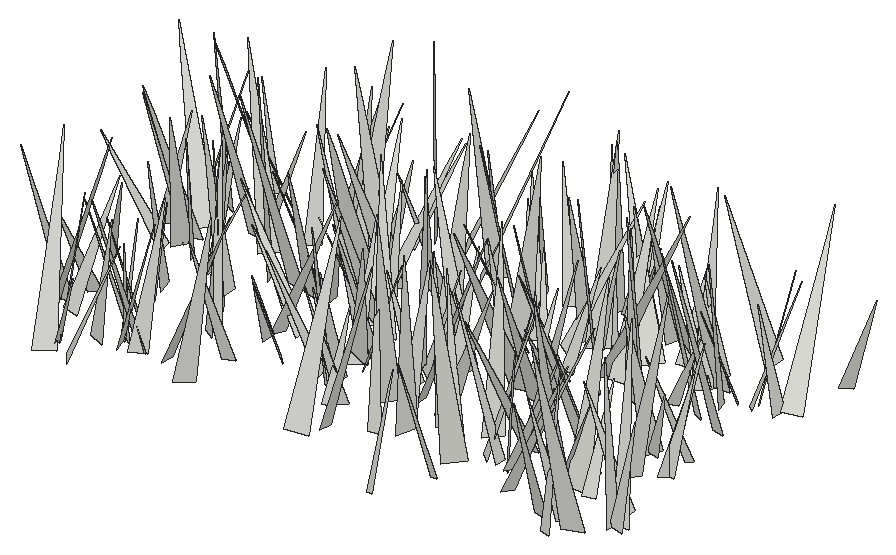
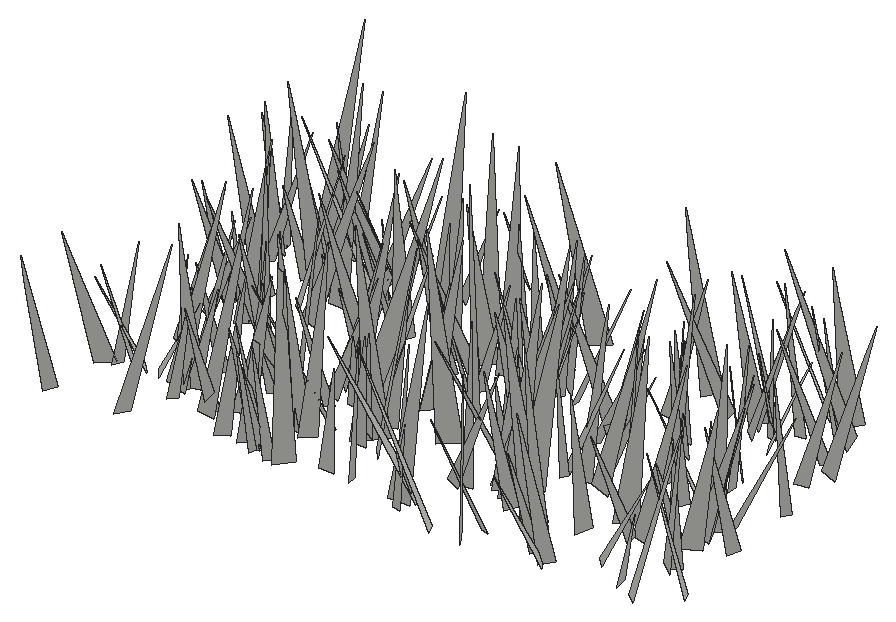
# SketchUp Ruby script. Lengths in inches.
U = 1.inch
M = Sketchup.active_model
def pt(a) = Geom::Point3d.new(a.map { |v| v * U })
def face(e, loops, mat)
  f = e.add_face(loops[0].map { |a| pt(a) })
  loops[1..].each { |l| e.add_face(l.map { |a| pt(a) }).erase! }
  f.material = f.back_material = mat if mat
  f
end
# faces: each face lists its corners as indices into pts; further lists are holes
def faces(e, pts, list, mat = nil) = list.each { |f| face(e, (f[0].is_a?(Array) ? f : [f]).map { |l| l.map { |i| pts[i] } }, mat) }
# xy, xz, yz: faces in a plane at the given z, y or x. An outline is a flat list of corners, or four numbers for a rectangle; further outlines are holes
def ring(l) = l.size == 4 ? [[l[0], l[1]], [l[2], l[1]], [l[2], l[3]], [l[0], l[3]]] : l.each_slice(2).to_a
def flat(e, list, mat, &to3) = list.each { |f| face(e, (f[0].is_a?(Array) ? f : [f]).map { |l| ring(l).map { |u, v| to3.(u, v) } }, mat) }
def xy(e, z, list, mat = nil) = flat(e, list, mat) { |x, y| [x, y, z] }
def xz(e, y, list, mat = nil) = flat(e, list, mat) { |x, z| [x, y, z] }
def yz(e, x, list, mat = nil) = flat(e, list, mat) { |y, z| [x, y, z] }
def lines(e, pts, list) = list.each { |a, b| e.add_line(pt(pts[a]), pt(pts[b])) }
# prism: a flat outline (further loops are holes) pulled along v
def prism(e, loops, v, mat = nil)
  f = face(e, loops, mat); d = Geom::Vector3d.new(v.map { |x| x * U })
  f.pushpull(f.normal.samedirection?(d) ? d.length : -d.length)
end
def box(e, o, s, mat = nil) = prism(e, [[o, [o[0] + s[0], o[1], o[2]], [o[0] + s[0], o[1] + s[1], o[2]], [o[0], o[1] + s[1], o[2]]]], [0, 0, s[2]], mat)
def at(x, y, z, deg = 0) = Geom::Transformation.translation(pt([x, y, z])) * Geom::Transformation.rotation(ORIGIN, Z_AXIS, deg.degrees)
def axes(o, x, y, z) = Geom::Transformation.new([*x, 0, *y, 0, *z, 0, *pt(o).to_a, 1])
def part(name) = M.definitions.add(name)
# library, detail: a bought-in or finely detailed component or shape, given as its bounding box
def library(name, o, s) = part(name).tap { |d| box(d.entities, o, s) }
def detail(e, o, s) = box(e.add_group.entities, o, s)
def put(e, d, t, mat = nil) = e.add_instance(d, t).tap { |i| i.material = mat if mat }
def group(e, t, mat = nil) = e.add_group.tap { |g| g.transformation = t; g.material = mat if mat }.entities
root = M.entities
c1 = part("fur_instance\#9")
p = [[0.8125,0,1.79],[0.67,-0.02,1.48],[0,-0.11,0],[0,0.11,0]]
faces(c1.entities,p,[[0,1,2,3]])
put(root,c1,axes([532.74,130.88,-21.66],[1.96135,3.70682,0.36248],[3.45553,-1.96392,1.38604],[-1.38968,0.34826,3.95807]))
put(root,c1,axes([503.99,133.75,-21.66],[3.91302,0.34843,0.25725],[0.41449,-3.69091,-1.30566],[-0.12562,-1.32482,3.70519]))
put(root,c1,axes([505.79,132.53,-21.66],[4.04604,3.23344,0.3968],[3.2461,-3.94826,-0.92578],[0.27467,-0.96906,5.09593]))
put(root,c1,axes([546.5,135.29,-21.66],[1.61042,-7.88282,1.5376],[-7.97737,-1.75156,-0.62458],[-0.92985,1.37466,8.02136]))
put(root,c1,axes([543.62,135.5,-21.66],[-0.77388,-5.77446,0.46112],[-5.72229,0.83441,0.84559],[0.90132,0.33953,5.76439]))
put(root,c1,axes([503.95,132.42,-21.66],[-5.29033,5.65073,1.03717],[5.57546,5.38985,-0.92613],[1.38587,-0.11308,7.68509]))
put(root,c1,axes([513.87,134.89,-21.66],[5.12868,-4.19399,1.94705],[-4.5125,-5.17419,0.74098],[-1.00889,1.82269,6.58361]))
put(root,c1,axes([545.2,135.82,-21.66],[0.47741,-4.86513,1.33169],[-4.92648,-0.73691,-0.92606],[-1.08291,1.20759,4.79999]))
put(root,c1,axes([534.81,135.12,-21.66],[0.7235,3.49331,2.20248],[3.65755,-1.58024,1.30491],[-1.91742,-1.69623,3.32022]))
put(root,c1,axes([505.73,135.68,-21.66],[-0.80392,-5.00028,1.94874],[-5.12712,1.2977,1.21465],[1.58527,1.66129,4.91668]))
put(root,c1,axes([503.87,134.27,-21.66],[4.42151,2.80893,1.55928],[2.73673,-4.68252,0.67492],[-1.68278,-0.23477,5.19464]))
put(root,c1,axes([545.27,133.86,-21.66],[2.35955,4.93164,1.36493],[4.86886,-2.62618,1.07189],[-1.57426,-0.73054,5.36093]))
put(root,c1,axes([502.5,134.3125,-21.66],[7.43833,2.19546,1.23858],[2.06036,-7.51855,0.95355],[-1.45225,0.57818,7.69672]))
put(root,c1,axes([509.09,136.38,-21.66],[-2.70694,-4.99144,1.16007],[-5.08628,2.45713,-1.29614],[-0.62448,1.62351,5.52829]))
put(root,c1,axes([507.4,136.17,-21.66],[5.27684,1.71083,0.85913],[1.8324,-5.24307,-0.81398],[-0.55438,-1.04563,5.4872]))
put(root,c1,axes([523.9,134.1875,-21.66],[-2.77927,7.20298,1.80131],[7.21654,3.07297,-1.15349],[1.74623,-1.2353,7.63392]))
put(root,c1,axes([507.19,137.08,-21.66],[-1.65671,-3.63214,1.3485],[-3.6613,1.94738,0.7471],[1.26719,0.87797,3.92161]))
put(root,c1,axes([534.58,137.59,-21.66],[4.88048,-6.02987,2.56967],[-6.14977,-5.32095,-0.80587],[-2.26779,1.4525,7.7155]))
put(root,c1,axes([508.95,136.0625,-21.66],[3.9195,-3.82723,2.46639],[-4.43668,-3.94163,0.93419],[-1.02305,2.43088,5.39791]))
put(root,c1,axes([548.6875,137.11,-21.66],[0.22976,-4.49295,1.68417],[-4.67204,0.17468,1.10336],[1.09322,1.69077,4.36142]))
put(root,c1,axes([524.9375,135.9375,-21.66],[6.05583,0.88682,1.38397],[0.67013,-6.15634,1.01257],[-1.50092,0.82941,6.03608]))
put(root,c1,axes([508.51,137.63,-21.66],[-2.89225,-3.68575,0.79235],[-3.76683,2.78458,-0.79678],[-0.15371,1.11313,4.61682]))
put(root,c1,axes([511.09,136.54,-21.66],[6.06997,0.80019,0.53139],[0.73411,-6.05703,0.73529],[-0.61948,0.66277,6.07817]))
put(root,c1,axes([539.79,136.8125,-21.66],[5.54197,-0.978,0.47716],[-1.05474,-5.437,1.10644],[-0.26776,1.17482,5.51777]))
put(root,c1,axes([514.28,139.09,-21.66],[0.3349,-5.08877,0.86463],[-5.08924,-0.4702,-0.79617],[-0.86188,0.79915,5.03725]))
put(root,c1,axes([529.61,138.8,-21.66],[6.66168,-2.88093,2.18206],[-2.80757,-7.00677,-0.67958],[-2.27567,0.211,7.22605]))
put(root,c1,axes([500.96,138.7,-21.66],[-1.48365,-5.76059,1.44193],[-5.8771,1.21156,-1.20691],[-0.85046,1.67706,5.82486]))
put(root,c1,axes([548.28,137.3,-21.66],[-5.81537,-0.03657,1.70774],[-0.23888,6.01751,-0.6846],[1.69135,0.72416,5.77505]))
put(root,c1,axes([507.2,136.69,-21.66],[1.88548,3.67223,0.79609],[3.49899,-2.04056,1.12569],[-1.36969,-0.15771,3.97154]))
put(root,c1,axes([523.89,139.15,-21.66],[0.22156,-4.52657,1.23949],[-4.53883,-0.5223,-1.09609],[-1.19379,1.1457,4.39744]))
put(root,c1,axes([548.08,139.21,-21.66],[-5.1344,0.67452,1.09766],[0.89094,5.11676,1.02317],[0.93062,-1.17714,5.07643]))
put(root,c1,axes([506.37,138.3,-21.66],[-4.07706,-2.14403,0.24298],[-2.12817,3.90987,-1.20919],[-0.35608,1.18084,4.44491]))
put(root,c1,axes([501.99,137.625,-21.66],[0.82135,5.31818,1.14764],[5.3338,-0.55827,-1.23031],[1.07271,-1.29616,5.2387]))
put(root,c1,axes([501.57,140.76,-21.66],[1.96703,-4.29578,0.10046],[-4.18734,-1.94112,-1.01553],[-0.96439,-0.33368,4.61429]))
put(root,c1,axes([527.99,137.38,-21.66],[0.38602,5.6901,1.15392],[5.67114,-0.61727,1.14668],[-1.24374,-1.04858,5.58671]))
put(root,c1,axes([523.28,138.38,-21.66],[-1.54021,3.23682,1.39983],[3.28512,1.87235,-0.71486],[1.28237,-0.90889,3.51258]))
put(root,c1,axes([540.67,141.06,-21.66],[-0.69616,-7.71222,1.47846],[-7.81205,0.83092,0.65597],[0.79755,1.40715,7.71575]))
put(root,c1,axes([541.72,140.1875,-21.66],[4.55769,0.07164,0.01251],[0.0727,-4.46545,-0.91231],[0.00209,-0.91239,4.46602]))
put(root,c1,axes([548.7,137.59,-21.66],[0.5538,7.06628,1.29605],[7.05626,-0.7792,1.23321],[-1.34954,-1.17443,6.97985]))
put(root,c1,axes([538.15,139.1,-21.66],[4.95013,-1.23925,0.4471],[-1.29852,-4.88303,0.8422],[-0.22245,0.9272,5.03291]))
put(root,c1,axes([537.6,141.98,-21.66],[0.04578,-6.29285,0.19538],[-6.21134,-0.07706,-1.02644],[-1.02831,0.18529,6.20874]))
put(root,c1,axes([526.07,141.1875,-21.66],[5.79688,-5.3049,1.7816],[-5.31494,-6.02201,-0.63769],[-1.75142,0.71643,7.83193]))
put(root,c1,axes([538.76,139.36,-21.66],[6.16739,3.42449,0.19717],[3.4017,-6.05394,-1.25736],[0.441,-1.19388,6.94138]))
put(root,c1,axes([522.88,139.65,-21.66],[0.28684,-3.45624,1.82339],[-3.70035,-0.82791,-0.9872],[-1.25608,1.64973,3.32465]))
put(root,c1,axes([521.8,141.41,-21.66],[4.64418,-2.47093,1.08294],[-2.19439,-4.71399,-1.3452],[-1.56935,-0.72073,5.0857]))
put(root,c1,axes([538.14,138.83,-21.66],[2.54415,2.86578,1.34064],[2.68524,-2.86561,1.02977],[-1.67317,-0.2414,3.6912]))
put(root,c1,axes([517.02,141.27,-21.66],[-2.4025,-2.92839,0.44923],[-2.80853,2.4353,0.85486],[0.94311,-0.20767,3.69008]))
put(root,c1,axes([536.98,139.47,-21.66],[-5.93557,-1.05009,0.32847],[-1.08922,5.86272,-0.94003],[0.15548,0.98355,5.95399]))
put(root,c1,axes([511.06,140.98,-21.66],[-1.26744,-3.38882,1.28492],[-3.35573,1.6115,0.94004],[1.36901,0.81271,3.49382]))
put(root,c1,axes([520.22,141.51,-21.66],[-4.86082,-0.82699,0.28427],[-0.77768,4.82218,0.73078],[0.39992,-0.67448,4.87621]))
put(root,c1,axes([543.32,139.77,-21.66],[-0.77106,7.66776,2.67234],[8.04873,1.0768,-0.76736],[1.07416,-2.56446,7.66813]))
put(root,c1,axes([521.7,140.36,-21.66],[-3.13424,-4.33981,2.11732],[-4.81159,3.01955,-0.93345],[0.40688,2.2779,5.27125]))
put(root,c1,axes([544.48,139.48,-21.66],[-1.99149,3.68652,0.84504],[3.6319,2.13053,-0.73532],[1.05538,-0.37542,4.12502]))
put(root,c1,axes([542.64,142.94,-21.66],[-3.72414,-4.2026,0.59605],[-4.10843,3.76818,0.89886],[1.06672,-0.15915,5.54285]))
put(root,c1,axes([527.93,140.9375,-21.66],[3.39124,-4.48702,2.29298],[-4.9912,-3.37077,0.78574],[-0.69206,2.32297,5.56924]))
put(root,c1,axes([535.83,139.36,-21.66],[3.94824,4.29759,0.4959],[4.2386,-3.97723,0.72087],[-0.86569,0.12707,5.79122]))
put(root,c1,axes([531.21,140.71,-21.66],[-0.70822,-5.57958,3.0516],[-6.3293,0.31925,-0.88519],[-0.61961,3.1164,5.55425]))
put(root,c1,axes([532.92,139.91,-21.66],[-5.60196,1.71083,0.59088],[1.59688,5.57635,-1.00614],[0.85208,0.79713,5.77032]))
put(root,c1,axes([514.48,143.01,-21.66],[3.47774,-1.50181,0.39234],[-1.2719,-3.30895,-1.39185],[-0.88975,-1.13996,3.5232]))
put(root,c1,axes([530.15,142.17,-21.66],[5.34451,-3.5502,0.35957],[-3.55754,-5.25077,1.03462],[0.27778,1.05952,6.33224]))
put(root,c1,axes([505.1,142.65,-21.66],[2.93725,2.51058,1.33666],[2.80043,-2.8887,-0.72813],[-0.49727,-1.43859,3.79478]))
put(root,c1,axes([540.76,143.98,-21.66],[-1.61608,-6.86234,1.14057],[-6.89566,1.42577,-1.19223],[-0.91789,1.37106,6.94853]))
put(root,c1,axes([521.15,144.21,-21.66],[2.32461,-5.72045,0.33614],[-5.68592,-2.25756,0.90225],[0.71192,0.64824,6.10846]))
put(root,c1,axes([534.47,141.875,-21.66],[-6.2785,3.87073,1.88034],[3.7817,6.55006,-0.85632],[2.05354,-0.22787,7.32591]))
put(root,c1,axes([504.8,144.11,-21.66],[-4.71927,-1.33587,1.95814],[-1.09743,5.09822,0.83318],[2.10107,-0.33763,4.83341]))
put(root,c1,axes([499.81,144.6,-21.66],[4.41728,-0.60705,0.29796],[-0.51929,-4.30631,-1.07505],[-0.43316,-1.02804,4.32726]))
put(root,c1,axes([521.92,144.01,-21.66],[4.65437,1.55789,0.49043],[1.62302,-4.57734,-0.86283],[-0.1826,-0.97553,4.83174]))
put(root,c1,axes([526.16,144.27,-21.66],[-4.20728,0.83557,0.99678],[1.00115,4.23485,0.67581],[0.83033,-0.87227,4.23588]))
put(root,c1,axes([534.18,142.87,-21.66],[4.3038,1.80689,1.01933],[1.67441,-4.41138,0.75005],[-1.22483,0.31842,4.60705]))
put(root,c1,axes([510.49,142.34,-21.66],[0.64289,6.12986,1.03372],[6.0316,-0.86662,1.38779],[-1.50455,-0.85491,6.00521]))
put(root,c1,axes([545.08,143.32,-21.66],[6.61649,-1.70465,2.3436],[-2.13195,-6.81989,1.0584],[-1.96294,1.66119,6.75008]))
put(root,c1,axes([515.89,144.79,-21.66],[-4.18794,0.93567,0.33129],[0.9893,4.05153,1.06324],[0.08071,-1.11073,4.15738]))
put(root,c1,axes([514.51,143.98,-21.66],[6.16079,-1.33707,0.34037],[-1.37023,-6.11166,0.79308],[-0.16154,0.84778,6.25413]))
put(root,c1,axes([527.73,142.68,-21.66],[6.18202,1.83786,0.77531],[1.68935,-6.16651,1.14736],[-1.06062,0.8903,6.34654]))
put(root,c1,axes([521.85,145.25,-21.66],[-1.08629,-5.09453,1.21583],[-5.17343,0.84989,-1.06105],[-0.81738,1.39139,5.09985]))
put(root,c1,axes([533.82,147.33,-21.66],[-0.13701,-6.93499,0.01519],[-6.899,0.13785,0.70555],[0.70571,0.00117,6.90036]))
put(root,c1,axes([509.59,144.35,-21.66],[4.32475,3.25099,2.86901],[3.37923,-5.06616,0.64681],[-2.71679,-1.12634,5.37159]))
put(root,c1,axes([532.06,148.03,-21.66],[1.01288,-8.11783,0.06805],[-8.08119,-1.01477,-0.77093],[-0.77341,-0.02823,8.14437]))
put(root,c1,axes([529.11,143.83,-21.66],[4.10356,-2.98524,2.70877],[-3.77942,-4.1935,1.10399],[-1.40181,2.56732,4.95298]))
put(root,c1,axes([544.13,146.71,-21.66],[4.71186,-4.25626,1.34995],[-4.06485,-4.9009,-1.26409],[-1.848,-0.07223,6.22249]))
put(root,c1,axes([546.75,145.02,-21.66],[-0.57371,3.97778,1.97621],[4.19128,1.14438,-1.08668],[1.47014,-1.71025,3.86924]))
put(root,c1,axes([508.65,145.89,-21.66],[-6.63003,0.58928,2.6026],[0.94805,7.03587,0.82207],[2.49439,-1.10786,6.6052]))
put(root,c1,axes([521.1875,143.93,-21.66],[-4.05743,3.11883,1.27429],[2.94276,4.25195,-1.03673],[1.64046,0.08657,5.0115]))
put(root,c1,axes([544.29,146.55,-21.66],[0.84418,-3.62493,0.18375],[-3.45271,-0.74384,1.18829],[1.11924,0.43944,3.52714]))
put(root,c1,axes([535.8,144.41,-21.66],[6.16496,0.12051,1.82007],[-0.27856,-6.27765,1.3592],[-1.80266,1.38221,6.01447]))
put(root,c1,axes([524.73,146.41,-21.66],[4.42565,6.01002,3.52258],[6.87552,-4.43985,-1.06317],[-1.12079,-3.50468,7.38759]))
put(root,c1,axes([525.68,145.6875,-21.66],[2.6257,3.60497,0.95618],[3.72031,-2.44904,-0.98281],[0.26337,-1.34567,4.35019]))
put(root,c1,axes([546.72,144.8,-21.66],[4.55494,-1.38322,1.77977],[-1.90749,-4.50337,1.38185],[-1.20098,1.9065,4.55536]))
put(root,c1,axes([527.64,147.8125,-21.66],[2.72704,-3.27265,0.76108],[-3.17295,-2.83078,-0.80329],[-1.10537,0.05182,4.1835]))
put(root,c1,axes([546.74,147.35,-21.66],[-0.5806,-4.0301,0.94816],[-3.96701,0.26756,-1.29192],[-1.18471,1.07913,3.86131]))
put(root,c1,axes([506.03,147.81,-21.66],[5.48101,-1.25937,0.85366],[-1.15676,-5.52263,-0.72019],[-0.98826,-0.52035,5.57753]))
put(root,c1,axes([505.86,146.375,-21.66],[3.45283,2.51437,0.03768],[2.48973,-3.40925,-0.65094],[0.3531,-0.54815,4.22141]))
put(root,c1,axes([501.48,148.26,-21.66],[-4.90231,-0.23018,0.15933],[-0.18525,4.76264,1.18065],[0.20988,-1.17272,4.76358]))
put(root,c1,axes([512.93,147.22,-21.66],[-4.21656,2.08304,0.19454],[2.06998,4.09043,1.06765],[-0.30342,-1.04195,4.58024]))
put(root,c1,axes([518.06,149.06,-21.66],[-3.59271,-3.52154,0.36411],[-3.38524,3.56898,1.11534],[1.03633,-0.55007,4.90559]))
put(root,c1,axes([513.2,149.23,-21.66],[-0.67207,-6.04885,0.74296],[-6.03248,0.76649,0.78356],[0.86591,0.6451,6.03542]))
put(root,c1,axes([519.13,148.76,-21.66],[-0.74587,-6.40704,1.23448],[-6.45249,0.53969,-1.09751],[-0.96927,1.33753,6.35625]))
put(root,c1,axes([534.17,149.13,-21.66],[1.81992,-3.21241,0.00061],[-3.09433,-1.75321,-0.99152],[-0.86298,-0.48823,3.55649]))
put(root,c1,axes([502.11,149.27,-21.66],[4.76035,-4.27512,0.72339],[-4.20428,-4.81383,-0.78223],[-1.06017,-0.10597,6.35025]))
put(root,c1,axes([519.03,147.21,-21.66],[-7.32876,-0.97242,0.83606],[-1.07916,7.29688,-0.97277],[0.69283,1.07947,7.32872]))
put(root,c1,axes([511.65,149.59,-21.66],[-2.25691,-7.5793,1.44794],[-7.71352,2.17504,-0.63772],[-0.20948,1.56823,7.88243]))
put(root,c1,axes([515.05,148.67,-21.66],[-3.55918,-3.90599,0.48478],[-3.91702,3.45103,-0.95229],[-0.38568,0.99656,5.19785]))
put(root,c1,axes([527.17,148.06,-21.66],[-5.93712,3.87569,1.72238],[4.1151,5.9813,0.72589],[1.02637,-1.56207,7.0529]))
put(root,c1,axes([514.61,149.61,-21.66],[4.05285,-0.43746,0.41546],[-0.3233,-3.95717,-1.01285],[-0.50937,-0.96903,3.94856]))
put(root,c1,axes([501.86,150.01,-21.66],[-5.14482,-3.13912,1.24988],[-3.04737,5.29445,0.7535],[1.4594,-0.01101,5.97959]))
put(root,c1,axes([503.72,148.37,-21.66],[-3.72029,-1.54775,1.40082],[-1.82397,3.80239,-0.64288],[1.01535,1.15959,3.97778]))
put(root,c1,axes([520.62,147.79,-21.66],[-2.14866,5.91991,1.32548],[6.06222,2.04254,0.70466],[-0.22751,-1.48381,6.25824]))
put(root,c1,axes([533.73,149.1,-21.66],[-3.99562,-4.42007,1.47298],[-4.65768,3.83659,-1.12173],[0.11293,1.84803,5.85182]))
put(root,c1,axes([532.43,148.39,-21.66],[-0.05946,3.80591,1.08242],[3.88392,0.26301,-0.71143],[0.75616,-1.05166,3.7393]))
put(root,c1,axes([515.28,152.35,-21.66],[4.78768,-6.87101,0.53821],[-6.76798,-4.81092,-1.21319],[-1.30189,-0.25808,8.28619]))
put(root,c1,axes([502.28,150.49,-21.66],[-0.64276,-5.9949,1.38637],[-6.03632,0.34404,-1.31091],[-1.1932,1.48889,5.88502]))
put(root,c1,axes([533.38,150.77,-21.66],[-0.33962,-4.53633,0.58104],[-4.49375,0.22275,-0.88758],[-0.84975,0.63509,4.46159]))
put(root,c1,axes([509.49,149.45,-21.66],[-6.31517,-2.67121,2.41272],[-3.08957,6.52254,-0.86542],[1.84694,1.77736,6.80204]))
put(root,c1,axes([528.45,152.8,-21.66],[-3.25593,-5.45811,0.05054],[-5.36708,3.21208,1.12765],[0.99394,-0.53501,6.25464]))
put(root,c1,axes([539.3,151.46,-21.66],[-3.95013,-6.45103,2.53754],[-6.55598,4.42551,1.04517],[2.25256,1.56763,7.49179]))
put(root,c1,axes([538.61,151.38,-21.66],[-1.6159,-6.90986,2.38073],[-7.13771,2.01606,1.00679],[1.57067,2.05292,7.0245]))
put(root,c1,axes([527.76,151.75,-21.66],[3.7662,-3.06911,1.25827],[-2.92554,-3.97067,-0.92842],[-1.56328,0.03677,4.76883]))
put(root,c1,axes([523.4,150.83,-21.66],[-3.8242,6.03816,3.67075],[6.53219,4.61268,-0.78232],[2.69524,-2.61192,7.10435]))
put(root,c1,axes([499.39,150.73,-21.66],[4.23339,-1.74729,1.15695],[-1.93705,-4.25778,0.65751],[-0.79963,1.0637,4.53236]))
put(root,c1,axes([518.63,148.56,-21.66],[-3.78371,6.02543,0.57396],[5.96039,3.82698,-0.88298],[1.05307,-0.01122,7.05993]))
put(root,c1,axes([545.73,151.64,-21.66],[-2.90009,-5.61636,1.60668],[-5.82709,2.65472,-1.23809],[-0.41218,1.98605,6.19848]))
put(root,c1,axes([535.98,151.14,-21.66],[3.85266,4.81198,3.39076],[5.17881,-4.69725,0.78179],[-2.79863,-2.06788,6.11449]))
put(root,c1,axes([516.89,153.52,-21.66],[1.34944,-6.66989,1.0863],[-6.57389,-1.5523,-1.36482],[-1.56569,0.76902,6.66676]))
put(root,c1,axes([505.28,153.25,-21.66],[-1.29627,-6.42722,1.30707],[-6.54569,1.18361,-0.67151],[-0.41416,1.4099,6.52216]))
put(root,c1,axes([516.8,153.77,-21.66],[3.0521,-3.8403,0.46149],[-3.78154,-3.08617,-0.67208],[-0.8129,-0.06212,4.85917]))
put(root,c1,axes([541.03,152.71,-21.66],[2.68666,-2.71893,0.01615],[-2.65256,-2.616,0.85524],[0.59729,0.61233,3.72549]))
put(root,c1,axes([543.38,152.45,-21.66],[-3.32572,-4.76152,1.64129],[-5.0351,3.09772,-1.21581],[-0.11678,2.03921,5.67929]))
put(root,c1,axes([531.47,150.94,-21.66],[-0.67642,4.08917,0.12939],[3.98053,0.62749,0.97839],[-0.94522,-0.2838,4.0276]))
put(root,c1,axes([507.39,152.11,-21.66],[3.71191,-5.65782,4.04126],[-6.28277,-4.69165,-0.79764],[-2.97818,2.84578,6.7196]))
put(root,c1,axes([518.24,151.23,-21.66],[-3.95695,1.67084,0.9926],[1.45221,4.03835,-1.00857],[1.29152,0.5783,4.17516]))
put(root,c1,axes([532.73,151.9,-21.66],[0.16923,4.07191,1.2027],[4.12697,0.12503,-1.00402],[0.99752,-1.2081,3.94982]))
put(root,c1,axes([527.45,153.38,-21.66],[5.01911,-5.50348,2.14134],[-5.83765,-5.04831,0.7082],[-0.89193,2.07156,7.41473]))
put(root,c1,axes([518.71,154.79,-21.66],[-0.89521,-5.51634,1.09126],[-5.41102,1.14576,1.35291],[1.53027,0.82431,5.42227]))
put(root,c1,axes([501.875,152.13,-21.66],[-4.84886,5.21937,0.60309],[5.25064,4.78392,0.8135],[-0.19034,-0.99462,7.07753]))
put(root,c1,axes([503.04,152,-21.66],[-3.70619,1.07071,1.22273],[0.63141,3.75399,-1.37341],[1.4976,1.06701,3.605]))
put(root,c1,axes([526.24,154.92,-21.66],[-5.36571,-5.00333,1.81378],[-4.95811,5.63559,0.87824],[1.93398,0.5664,7.28374]))
put(root,c1,axes([535.12,152.86,-21.66],[7.55011,-1.58138,0.22082],[-1.59514,-7.42262,1.38345],[0.0711,1.39915,7.58887]))
put(root,c1,axes([515.36,154.3,-21.66],[3.59874,-6.83955,3.08177],[-7.12327,-4.18751,-0.97538],[-2.35281,2.21652,7.66674]))
put(root,c1,axes([501.02,154.76,-21.66],[0.91273,-4.1627,0.50654],[-4.12867,-0.80133,0.85424],[0.734,0.66898,4.1751]))
put(root,c1,axes([516.92,152.19,-21.66],[2.4518,5.85296,0.01413],[5.81055,-2.43218,-0.76857],[0.70347,-0.30989,6.29903]))
put(root,c1,axes([531.23,156.08,-21.66],[5.68928,-3.36377,1.44998],[-3.11585,-5.85243,-1.35122],[-1.92583,-0.46842,6.46971]))
put(root,c1,axes([519.79,155,-21.66],[-0.88602,-4.48963,1.06047],[-4.46813,0.56653,-1.33464],[-1.14769,1.26043,4.37728]))
put(root,c1,axes([505.84,153.4375,-21.66],[4.17653,-0.25853,0.87813],[-0.4857,-4.1025,1.10224],[-0.77592,1.17643,4.03674]))
put(root,c1,axes([536.4,152.82,-21.66],[-1.26821,6.79621,1.34265],[6.86908,1.41065,-0.65215],[0.89826,-1.19212,6.8827]))
put(root,c1,axes([528.29,153.74,-21.66],[-1.05429,4.67357,0.99792],[4.75005,0.91265,0.74413],[-0.52453,-1.12891,4.73287]))
put(root,c1,axes([543.76,154.48,-21.66],[-4.56501,-1.69942,1.47091],[-1.97129,4.62695,-0.77219],[1.07964,1.26263,4.80947]))
put(root,c1,axes([514.65,155.21,-21.66],[3.82808,-2.96393,0.87418],[-3.08142,-3.76593,0.72521],[-0.23226,1.11183,4.78677]))
put(root,c1,axes([538.39,157.94,-21.66],[-2.04467,-7.63412,0.65301],[-7.56547,2.11851,1.07815],[1.21235,0.345,7.82931]))
put(root,c1,axes([542.29,156.28,-21.66],[-1.50167,-7.67594,2.08534],[-7.92089,1.24921,-1.10571],[-0.72669,2.24569,7.7429]))
put(root,c1,axes([501.56,155.1,-21.66],[-3.6941,-4.73944,2.34113],[-5.23892,3.66336,-0.85037],[0.70493,2.38895,5.94858]))
put(root,c1,axes([547.31,156.12,-21.66],[-4.17455,0.44699,1.70239],[0.80041,4.38471,0.81146],[1.56757,-1.04848,4.11925]))
put(root,c1,axes([544.33,155.53,-21.66],[-3.00148,-2.27694,0.1564],[-2.20162,2.82047,-1.1898],[-0.60148,1.03841,3.57459]))
put(root,c1,axes([532.32,155.95,-21.66],[2.08402,3.38406,1.47593],[3.68931,-1.84524,-0.97848],[0.13865,-1.76538,3.85196]))
put(root,c1,axes([541.26,155.66,-21.66],[-2.68831,3.38264,1.06218],[3.54497,2.54168,0.8778],[-0.06058,-1.37662,4.23069]))
put(root,c1,axes([530.9,153.9375,-21.66],[2.76171,5.55128,0.00194],[5.48471,-2.72826,-0.95829],[0.85713,-0.42855,6.1258]))
put(root,c1,axes([528.06,154.76,-21.66],[-1.29816,5.29172,0.79515],[5.27739,1.13069,1.0911],[-0.88529,-1.01932,5.33826]))
put(root,c1,axes([508.99,154.6,-21.66],[-5.25856,3.05312,1.43062],[2.8843,5.44607,-1.02073],[1.74617,0.1987,5.99435]))
put(root,c1,axes([510.94,156.76,-21.66],[0.6303,-6.24139,2.24897],[-6.57772,-0.29373,1.02832],[0.86396,2.31708,6.18828]))
put(root,c1,axes([512.25,155.8125,-21.66],[-3.47776,6.78239,3.15196],[7.08859,4.09761,-0.99596],[2.38486,-2.28893,7.55669]))
put(root,c1,axes([532.37,155.57,-21.66],[-5.26533,5.42334,2.66225],[5.51698,5.75546,-0.81326],[2.46233,-1.29842,7.51498]))
put(root,c1,axes([505.51,157.16,-21.66],[-2.7303,-2.91554,0.15676],[-2.8364,2.59761,-1.08937],[-0.69267,0.85529,3.84294]))
put(root,c1,axes([541.29,155.48,-21.66],[-5.91196,3.62871,1.99788],[3.48429,6.23911,-1.02156],[2.24027,-0.12769,6.86114]))
put(root,c1,axes([541.53,157.55,-21.66],[-3.71371,1.13934,1.58672],[1.47505,3.87017,0.67337],[1.28063,-1.15373,3.82574]))
put(root,c1,axes([498.09,157.37,-21.66],[4.56554,2.4835,0.72557],[2.58092,-4.47494,-0.92307],[-0.18188,-1.15993,5.11467]))
put(root,c1,axes([545.45,155.46,-21.66],[3.29969,3.36632,0.10349],[3.25213,-3.22241,1.12716],[-0.87548,0.71745,4.57707]))
put(root,c1,axes([532.77,156.4375,-21.66],[1.28068,6.67783,2.12971],[6.86225,-1.63556,1.00185],[-1.42781,-1.87102,6.72532]))
put(root,c1,axes([536.59,156.1875,-21.66],[-4.59485,5.55244,0.46156],[5.5505,4.50971,1.00485],[-0.48434,-0.99407,7.1367]))
put(root,c1,axes([535.84,159.39,-21.66],[4.30794,-3.29071,0.86204],[-3.07513,-4.36194,-1.28347],[-1.45447,-0.52435,5.26686]))
put(root,c1,axes([545.42,156.44,-21.66],[3.89268,2.82638,0.90518],[2.67493,-3.98806,0.94914],[-1.28551,0.26015,4.71599]))
put(root,c1,axes([500.9,159.76,-21.66],[-3.86726,-4.8383,0.71579],[-4.78645,3.93151,0.71436],[1.00566,0.10641,6.1526]))
put(root,c1,axes([534.05,159.17,-21.66],[4.56733,-2.95407,1.62637],[-2.80415,-4.84794,-0.93072],[-1.87305,0.05455,5.35918]))
put(root,c1,axes([525.3,158.85,-21.66],[-4.30625,-1.78107,2.16646],[-1.55574,4.81995,0.87021],[2.33354,-0.07334,4.57807]))
put(root,c1,axes([538.29,157.21,-21.66],[-1.13275,3.97734,1.11963],[3.98013,1.3621,-0.81189],[1.10966,-0.82546,4.05502]))
put(root,c1,axes([521.09,159.12,-21.66],[0.92373,-7.0899,2.33425],[-7.39568,-1.18748,-0.68009],[-1.00963,2.21177,7.11741]))
put(root,c1,axes([530.23,159.83,-21.66],[7.09602,-3.54407,1.49132],[-3.45875,-7.25092,-0.77408],[-1.67974,-0.04148,7.89397]))
put(root,c1,axes([520.56,159.97,-21.66],[-2.364,-4.99525,1.36106],[-4.8414,2.66304,1.36474],[1.83462,0.59091,5.35523]))
put(root,c1,axes([532.5,159.17,-21.66],[4.32257,0.5968,0.21737],[0.63053,-4.21214,-0.97382],[-0.07654,-0.99484,4.25352]))
put(root,c1,axes([508.21,159.5,-21.66],[4.08731,-3.32744,0.79787],[-3.41978,-4.01464,0.77613],[-0.11643,1.10699,5.21302]))
put(root,c1,axes([509.62,158.9,-21.66],[-0.91828,3.53646,1.4047],[3.57282,1.29857,-0.93362],[1.30946,-1.06309,3.53244]))
put(root,c1,axes([531.29,160.14,-21.66],[1.4619,-3.63585,0.57448],[-3.60479,-1.28901,1.01518],[0.74496,0.89757,3.78497]))
put(root,c1,axes([548.03,156.57,-21.66],[-3.4412,6.39637,0.09759],[6.32165,3.41718,-1.06042],[0.97968,0.41743,7.18546]))
put(root,c1,axes([502.64,158.59,-21.66],[-3.94683,-0.00707,0.27926],[-0.08275,3.80753,-1.07302],[0.26682,1.07619,3.79817]))
put(root,c1,axes([514.09,158.74,-21.66],[2.1149,3.97719,0.39309],[3.90996,-1.96694,-1.13523],[0.82754,-0.87089,4.35914]))
put(root,c1,axes([527.41,158.88,-21.66],[-1.32199,4.73147,0.88748],[4.77716,1.17578,0.84759],[-0.59431,-1.0737,4.83901]))
put(root,c1,axes([542.96,161.09,-21.66],[-6.41083,1.14128,1.69671],[1.48537,6.43646,1.28286],[1.40536,-1.59673,6.38401]))
put(root,c1,axes([520.5,157.93,-21.66],[5.97415,4.42308,0.10738],[4.35531,-5.91092,1.16532],[-0.77872,0.87356,7.3414]))
put(root,c1,axes([532.86,159.62,-21.66],[3.50267,-1.34823,2.1537],[-1.97697,-3.75014,0.86764],[-1.59615,1.68627,3.65152]))
put(root,c1,axes([532.64,159.49,-21.66],[-1.16488,5.07104,1.08343],[5.11451,1.30667,-0.61696],[0.85504,-0.90739,5.16641]))
put(root,c1,axes([548.65,161.63,-21.66],[3.25053,-3.28963,0.28157],[-3.26975,-3.15258,0.91484],[0.45796,0.84053,4.53329]))
put(root,c1,axes([517.09,160.77,-21.66],[5.75926,3.61485,0.22209],[3.58079,-5.62103,-1.36658],[0.54262,-1.27375,6.66098]))
put(root,c1,axes([514.87,160.3,-21.66],[-5.7993,-3.05465,2.69516],[-3.68736,5.92923,-1.21419],[1.7315,2.39584,6.44116]))
put(root,c1,axes([508.36,159.78,-21.66],[3.43862,2.40363,0.16823],[2.31203,-3.37399,0.94893],[-0.67841,0.6845,4.08669]))
